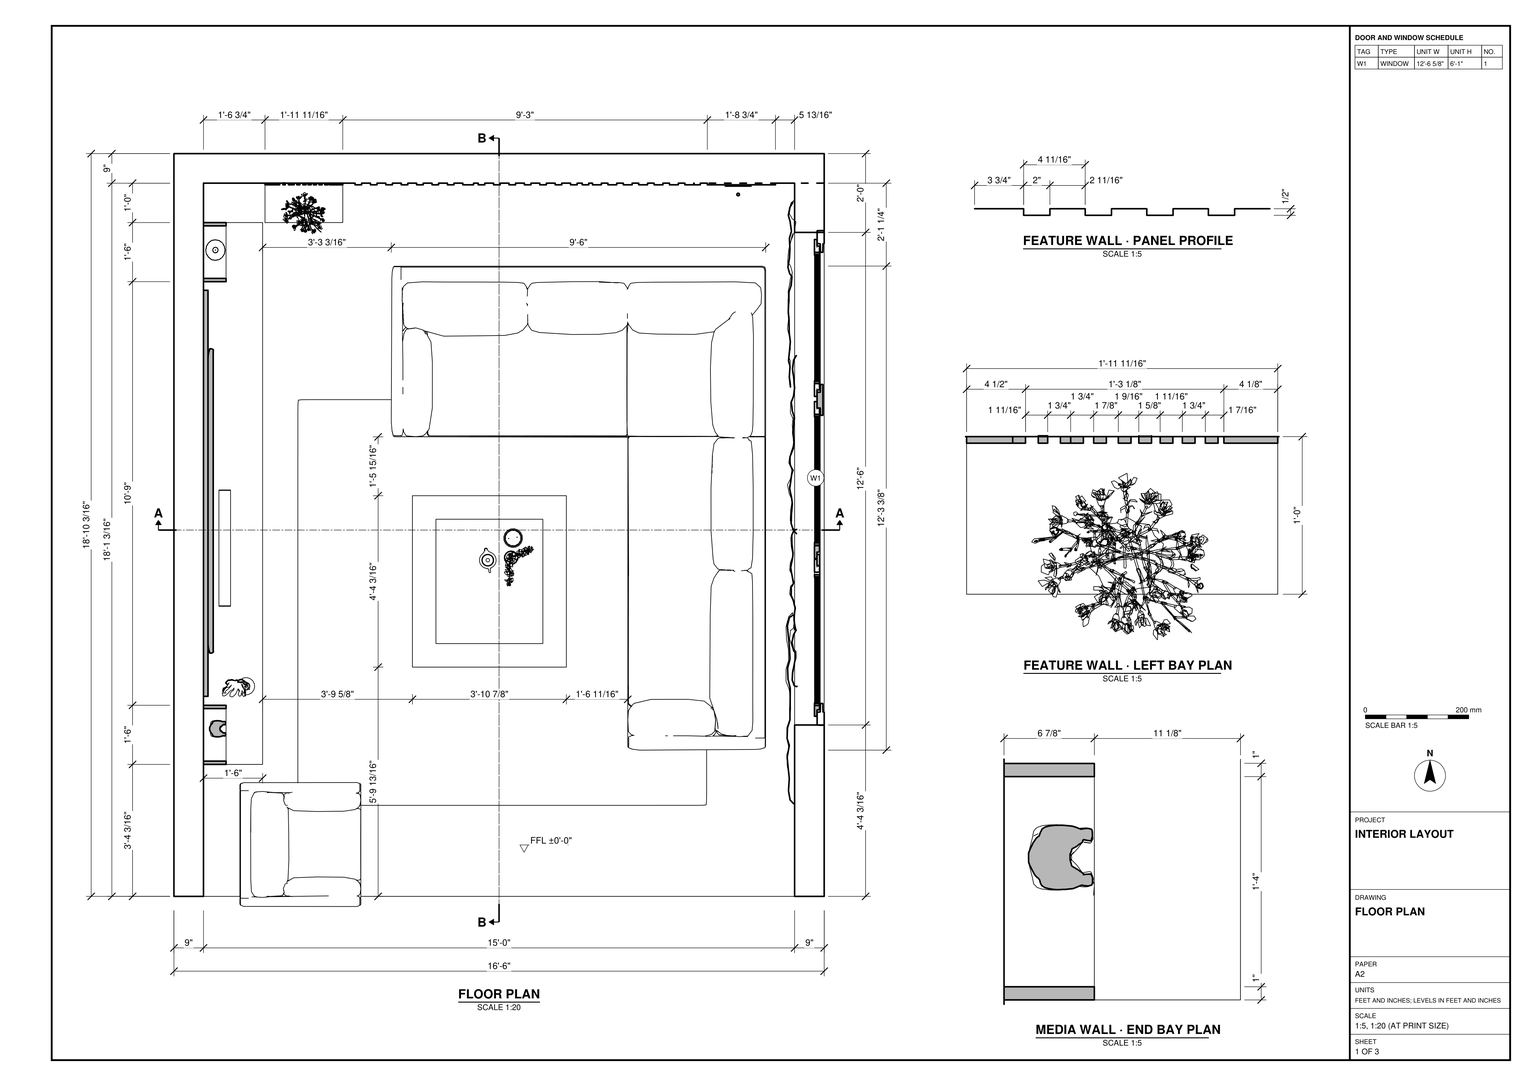
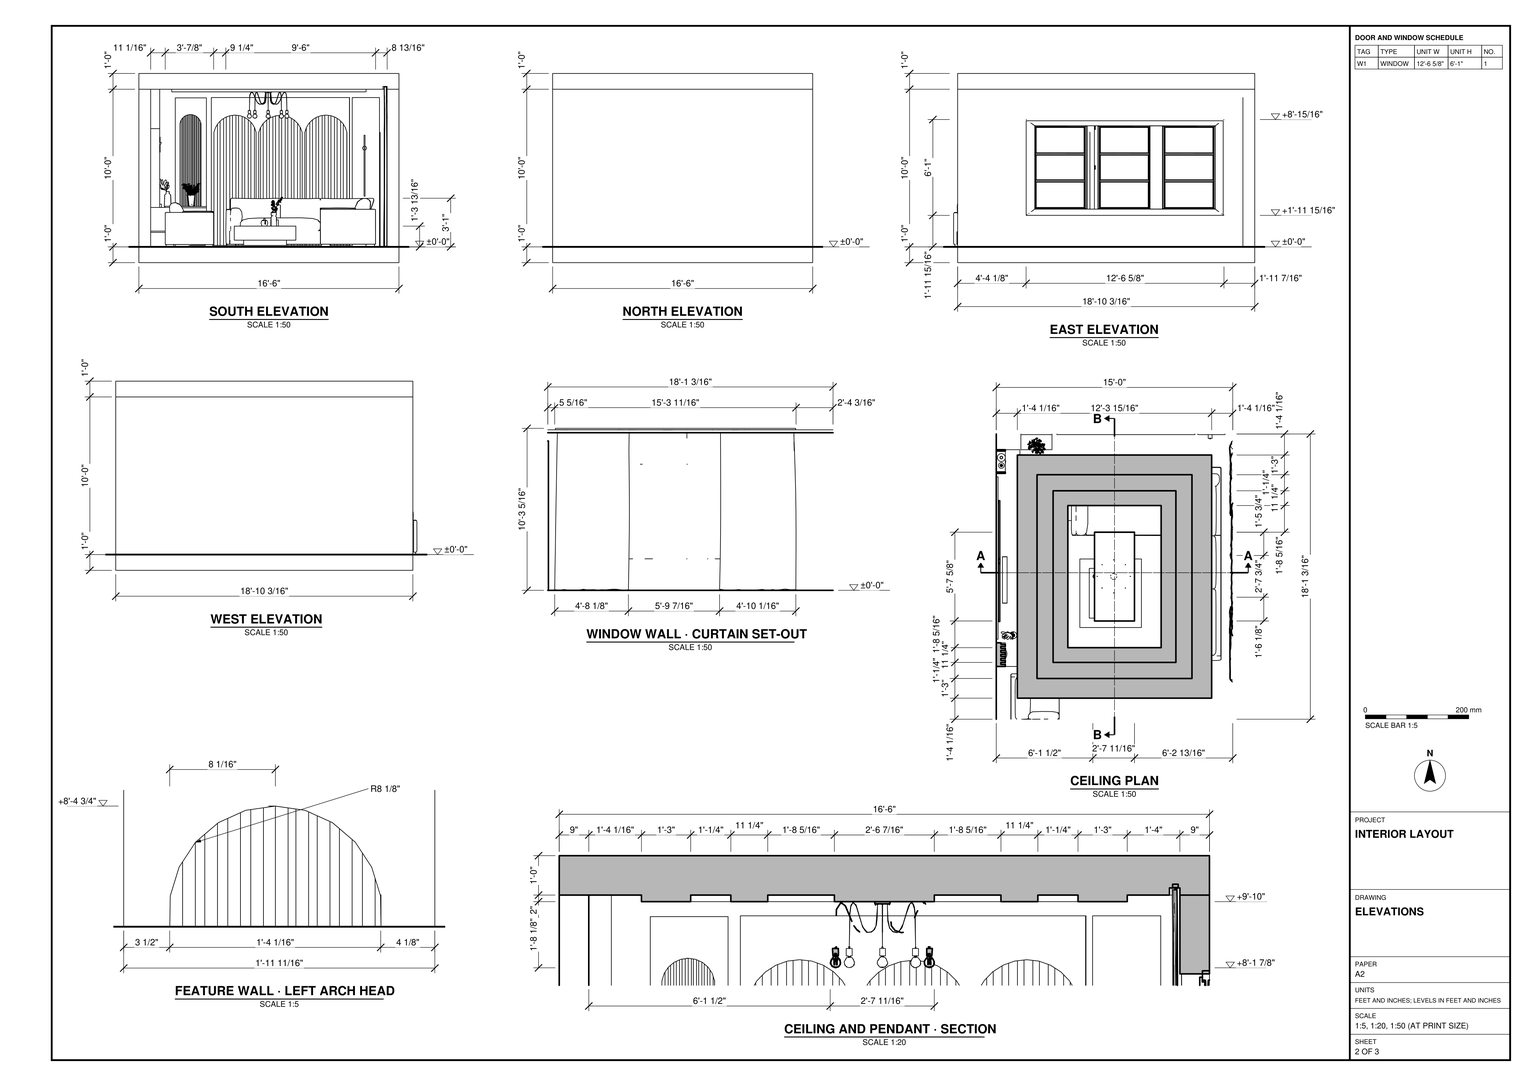
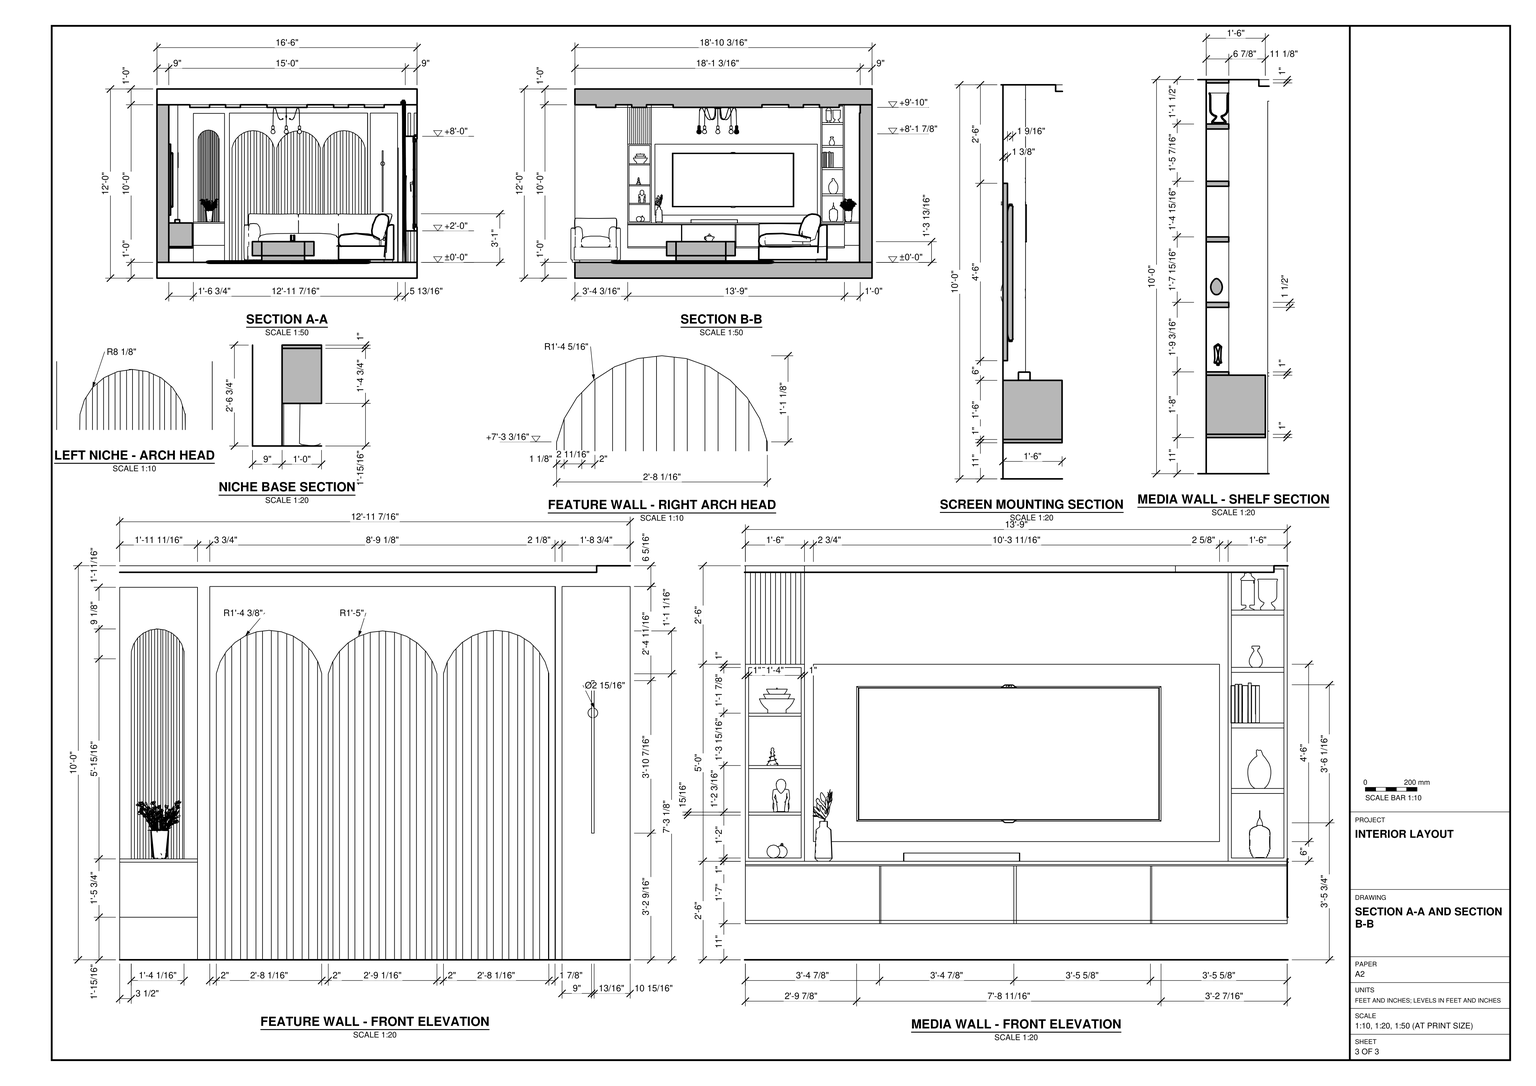
Build the furnished living room shown in task_files/diagram_01.pdf. Work in feet and inches. The overall model is 16'-6" wide, 19'-1 1/4" deep and 12'-0" high, with a single finished floor level at ±0'-0". Model the floor and ceiling slabs and the 9" walls on the north, east and west sides. Leave the south side open as drawn. Use the ceiling plan and sections to form the stepped rectangular bands overhead.

On the north wall, model the narrow arched display niche above its base, the three broad arches with vertical ribbing, and the plain end panel. On the west wall, build the low media cabinet with a screen on its backing panel and open shelves at both ends. Fit the divided window into the east wall and place the curtains on its room side.

Arrange the L-shaped sectional along the feature and window walls. Place the coffee table on the rug inside the L, the armchair near the open southwest corner and the pendant above the table. Decor and loose items may be any suitable library components.

Keep the shell elements and each furniture or joinery piece as separate groups or components, and use components for repeated parts. Save one SketchUp model as output_files/living_room_with_feature_and_media_walls.skp.

# SketchUp Ruby script. Lengths in inches.
U = 1.inch
M = Sketchup.active_model
def pt(a) = Geom::Point3d.new(a.map { |v| v * U })
def face(e, loops, mat)
  f = e.add_face(loops[0].map { |a| pt(a) })
  loops[1..].each { |l| e.add_face(l.map { |a| pt(a) }).erase! }
  f.material = f.back_material = mat if mat
  f
end
# faces: each face lists its corners as indices into pts; further lists are holes
def faces(e, pts, list, mat = nil) = list.each { |f| face(e, (f[0].is_a?(Array) ? f : [f]).map { |l| l.map { |i| pts[i] } }, mat) }
# xy, xz, yz: faces in a plane at the given z, y or x. An outline is a flat list of corners, or four numbers for a rectangle; further outlines are holes
def ring(l) = l.size == 4 ? [[l[0], l[1]], [l[2], l[1]], [l[2], l[3]], [l[0], l[3]]] : l.each_slice(2).to_a
def flat(e, list, mat, &to3) = list.each { |f| face(e, (f[0].is_a?(Array) ? f : [f]).map { |l| ring(l).map { |u, v| to3.(u, v) } }, mat) }
def xy(e, z, list, mat = nil) = flat(e, list, mat) { |x, y| [x, y, z] }
def xz(e, y, list, mat = nil) = flat(e, list, mat) { |x, z| [x, y, z] }
def yz(e, x, list, mat = nil) = flat(e, list, mat) { |y, z| [x, y, z] }
def lines(e, pts, list) = list.each { |a, b| e.add_line(pt(pts[a]), pt(pts[b])) }
# prism: a flat outline (further loops are holes) pulled along v
def prism(e, loops, v, mat = nil)
  f = face(e, loops, mat); d = Geom::Vector3d.new(v.map { |x| x * U })
  f.pushpull(f.normal.samedirection?(d) ? d.length : -d.length)
end
def box(e, o, s, mat = nil) = prism(e, [[o, [o[0] + s[0], o[1], o[2]], [o[0] + s[0], o[1] + s[1], o[2]], [o[0], o[1] + s[1], o[2]]]], [0, 0, s[2]], mat)
def at(x, y, z, deg = 0) = Geom::Transformation.translation(pt([x, y, z])) * Geom::Transformation.rotation(ORIGIN, Z_AXIS, deg.degrees)
def axes(o, x, y, z) = Geom::Transformation.new([*x, 0, *y, 0, *z, 0, *pt(o).to_a, 1])
def part(name) = M.definitions.add(name)
# library, detail: a bought-in or finely detailed component or shape, given as its bounding box
def library(name, o, s) = part(name).tap { |d| box(d.entities, o, s) }
def detail(e, o, s) = box(e.add_group.entities, o, s)
def put(e, d, t, mat = nil) = e.add_instance(d, t).tap { |i| i.material = mat if mat }
def group(e, t, mat = nil) = e.add_group.tap { |g| g.transformation = t; g.material = mat if mat }.entities
root = M.entities
M.materials.add("Delta-Grail-185LF-SS").color = [45, 45, 45]
c1 = library("Window 46-31",[-44.57,-2.6,0],[89.14,5.19,59.84])
c2 = library("Curtains 001",[-91.88,-6.87,0.16],[183.71,15.03,109.46])
c3 = library("Fairfax Sectional",[-59.93,-44.96,0],[104.54,100.01,33.05])
c4 = part("Группа\#472")
prism(c4.entities,[[[0.67,0.67,0],[0.73,0.59,0],[0.77,0.5,0],[0.79,0.39,0],[0.77,0.29,0],[0.73,0.2,0],[0.67,0.12,0],[0.59,0.05,0],[0.5,0.01,0],[0.39,0,0],[0.29,0.01,0],[0.2,0.05,0],[0.12,0.12,0],[0.05,0.2,0],[0.01,0.29,0],[0,0.39,0],[0.01,0.5,0],[0.05,0.59,0],[0.12,0.67,0],[0.2,0.73,0],[0.29,0.77,0],[0.39,0.79,0],[0.5,0.77,0],[0.59,0.73,0]]],[0,0,46.46],"Delta-Grail-185LF-SS")
c5 = part("Группа\#471")
prism(c5.entities,[[[2.95,2.79,0.8],[2.95,2.83,0.88],[2.95,2.86,0.97],[2.95,2.89,1.06],[2.95,2.92,1.15],[2.95,2.93,1.24],[2.95,2.95,1.33],[2.95,2.95,1.42],[2.95,2.95,1.52],[2.95,2.95,1.61],[2.95,2.93,1.7],[2.95,2.92,1.79],[2.95,2.9,1.88],[2.95,2.87,1.97],[2.95,2.83,2.06],[2.95,2.79,2.14],[2.95,2.75,2.22],[2.95,2.7,2.3],[2.95,2.65,2.375],[2.95,2.59,2.45],[2.95,2.52,2.52],[2.95,2.46,2.58],[2.95,2.38,2.64],[2.95,2.31,2.69],[2.95,2.23,2.74],[2.95,2.15,2.79],[2.95,2.07,2.83],[2.95,1.98,2.86],[2.95,1.89,2.89],[2.95,1.8,2.92],[2.95,1.71,2.93],[2.95,1.62,2.95],[2.95,1.53,2.95],[2.95,1.43,2.95],[2.95,1.34,2.95],[2.95,1.25,2.93],[2.95,1.16,2.92],[2.95,1.07,2.9],[2.95,0.98,2.87],[2.95,0.89,2.83],[2.95,0.81,2.79],[2.95,0.73,2.75],[2.95,0.65,2.7],[2.95,0.58,2.65],[2.95,0.5,2.59],[2.95,0.4375,2.52],[2.95,0.37,2.46],[2.95,0.3125,2.38],[2.95,0.26,2.31],[2.95,0.21,2.23],[2.95,0.16,2.15],[2.95,0.12,2.07],[2.95,0.09,1.98],[2.95,0.06,1.89],[2.95,0.04,1.8],[2.95,0.02,1.71],[2.95,0.01,1.62],[2.95,0,1.53],[2.95,0,1.43],[2.95,0.01,1.34],[2.95,0.02,1.25],[2.95,0.03,1.16],[2.95,0.06,1.07],[2.95,0.08,0.98],[2.95,0.12,0.89],[2.95,0.16,0.81],[2.95,0.2,0.73],[2.95,0.25,0.65],[2.95,0.31,0.58],[2.95,0.36,0.5],[2.95,0.43,0.4375],[2.95,0.5,0.37],[2.95,0.57,0.3125],[2.95,0.64,0.26],[2.95,0.72,0.21],[2.95,0.8,0.16],[2.95,0.88,0.12],[2.95,0.97,0.09],[2.95,1.06,0.06],[2.95,1.15,0.04],[2.95,1.24,0.02],[2.95,1.33,0.01],[2.95,1.42,0],[2.95,1.52,0],[2.95,1.61,0.01],[2.95,1.7,0.02],[2.95,1.79,0.03],[2.95,1.88,0.06],[2.95,1.97,0.08],[2.95,2.06,0.12],[2.95,2.14,0.16],[2.95,2.22,0.2],[2.95,2.3,0.25],[2.95,2.375,0.31],[2.95,2.45,0.36],[2.95,2.52,0.43],[2.95,2.58,0.5],[2.95,2.64,0.57],[2.95,2.69,0.64],[2.95,2.74,0.72]]],[-2.95,0,0],"Delta-Grail-185LF-SS")
c6 = part("KEMMA WALL L")
put(c6.entities,c4,at(0,1.08,0))
put(c6.entities,c5,at(0.39,0,35.14))
c7 = part("Группа\#357")
xy(c7.entities,0,[[0,0,118.11,15.75]])
c8 = part("Группа\#473")
put(c8.entities,c7,axes([0,7.84,0],[0,0,0.39176],[0,-0.25,0],[-1,0,0]))
put(c8.entities,c7,axes([0,0,0],[0,0,0.39176],[0,0.25,0],[1,0,0]))
c9 = part("Kemma wall")
put(c9.entities,c6,at(0,2.44,3.71))
put(c9.entities,c8,axes([2.95,0,0],[1,0,0],[0,1,0],[0,0,1.16295]))
c10 = library("Rug 293 007",[-90.2,-61.78,-0.71],[180.4,123.56,1.82])
c11 = library("Fairfax Chair",[-18.9,-18.43,0],[37.75,36.85,33.69])
c12 = library("TV Speaker 002",[-17.72,-1.77,0],[35.44,3.54,2.52])
c13 = library("download?mid=50c7180b9fccec56d493bfe20f94b6ab&ctyp=sp&cv=p8.",[149.43,43.83,17.86],[74.75,0.57,42.04])
c14 = library("Books 53-03",[-4.33,-4.86,0],[8.66,9.72,12.21])
c15 = library("Perfume 101 020",[-1.72,-1.72,-0.02],[3.44,3.44,5.4])
c16 = library("Perfume 101 004",[-2,-2,-0.02],[4,4,6.5])
c17 = library("Interior Props 221 031",[-3.74,-3.52,-0.04],[7.48,7.03,11.78])
c18 = library("Christmas Props 155 013 03",[-3.17,-3,-0.07],[6.8,6.18,4.48])
c19 = library("Interior Props 160 010",[-8.82,-8.31,0],[17.47,16.43,22.13])
c20 = library("Decorative Jar 83-09",[-5.58,-3.02,0],[11.21,6.04,13.74])
c21 = library("Fountain 108-01",[-21.4375,-21.4375,0],[42.875,42.875,30.71])
c22 = library("Decorative Jar 002",[-4.66,-4.66,0.02],[9.32,9.32,23.26])
c23 = library("Vase 007",[-9.22,-3.28,0],[11.85,5.91,21.89])
c24 = library("Interior Props 221 010",[-4.44,-3.51,-0.03],[8.89,7.03,15.76])
c25 = library("Vase 004",[-7.23,-6.39,-0.02],[13.74,12.68,17.81])
c26 = library("Pendant 81-14",[-15.9,-15.86,-20.15],[31.7,31.76,20.15])
xy(root,-12,[[0,0,198,226.1875]])
xy(root,0,[[0,0,9,0,9,217.1875,55.15,217.1875,55.15,216.6875,57.15,216.6875,57.15,217.1875,59.84,217.1875,59.84,216.6875,61.84,216.6875,61.84,217.1875,64.53,217.1875,64.53,216.6875,66.53,216.6875,66.53,217.1875,69.21,217.1875,69.21,216.6875,71.21,216.6875,71.21,217.1875,73.9,217.1875,73.9,216.6875,75.9,216.6875,75.9,217.1875,78.59,217.1875,78.59,216.6875,80.59,216.6875,80.59,217.1875,83.28,217.1875,83.28,216.6875,85.28,216.6875,85.28,217.1875,87.96,217.1875,87.96,216.6875,91.23,216.6875,91.23,217.1875,92.65,217.1875,92.65,216.6875,94.65,216.6875,94.65,217.1875,97.34,217.1875,97.34,216.6875,99.34,216.6875,99.34,217.1875,102.03,217.1875,102.03,216.6875,104.03,216.6875,104.03,217.1875,106.71,217.1875,106.71,216.6875,108.71,216.6875,108.71,217.1875,111.4,217.1875,111.4,216.6875,113.4,216.6875,113.4,217.1875,116.09,217.1875,116.09,216.6875,118.09,216.6875,118.09,217.1875,120.78,217.1875,120.78,216.6875,122.78,216.6875,122.78,217.1875,124.32,217.1875,124.32,216.6875,126.32,216.6875,126.32,217.1875,127.46,217.1875,127.46,216.6875,130.15,216.6875,130.15,217.1875,132.15,217.1875,132.15,216.6875,134.84,216.6875,134.84,217.1875,136.84,217.1875,136.84,216.6875,139.53,216.6875,139.53,217.1875,141.53,217.1875,141.53,216.6875,144.21,216.6875,144.21,217.1875,146.21,217.1875,146.21,216.6875,148.9,216.6875,148.9,217.1875,150.9,217.1875,150.9,216.6875,153.59,216.6875,153.59,217.1875,155.59,217.1875,155.59,216.6875,158.28,216.6875,158.28,217.1875,158.4,217.1875,158.4,216.6875,160.28,216.6875,160.28,217.1875,162.42,217.1875,162.42,216.6875,183.17,216.6875,183.17,217.1875,189,217.1875,189,0,198,0,198,226.1875,0,226.1875],[9,0,189,0,189,217.1875,183.17,217.1875,183.17,216.6875,162.42,216.6875,162.42,217.1875,160.28,217.1875,160.28,216.6875,158.4,216.6875,158.4,217.1875,158.28,217.1875,158.28,216.6875,155.59,216.6875,155.59,217.1875,153.59,217.1875,153.59,216.6875,150.9,216.6875,150.9,217.1875,148.9,217.1875,148.9,216.6875,146.21,216.6875,146.21,217.1875,144.21,217.1875,144.21,216.6875,141.53,216.6875,141.53,217.1875,139.53,217.1875,139.53,216.6875,136.84,216.6875,136.84,217.1875,134.84,217.1875,134.84,216.6875,132.15,216.6875,132.15,217.1875,130.15,217.1875,130.15,216.6875,127.46,216.6875,127.46,217.1875,126.32,217.1875,126.32,216.6875,124.32,216.6875,124.32,217.1875,122.78,217.1875,122.78,216.6875,120.78,216.6875,120.78,217.1875,118.09,217.1875,118.09,216.6875,116.09,216.6875,116.09,217.1875,113.4,217.1875,113.4,216.6875,111.4,216.6875,111.4,217.1875,108.71,217.1875,108.71,216.6875,106.71,216.6875,106.71,217.1875,104.03,217.1875,104.03,216.6875,102.03,216.6875,102.03,217.1875,99.34,217.1875,99.34,216.6875,97.34,216.6875,97.34,217.1875,94.65,217.1875,94.65,216.6875,92.65,216.6875,92.65,217.1875,91.23,217.1875,91.23,216.6875,87.96,216.6875,87.96,217.1875,85.28,217.1875,85.28,216.6875,83.28,216.6875,83.28,217.1875,80.59,217.1875,80.59,216.6875,78.59,216.6875,78.59,217.1875,75.9,217.1875,75.9,216.6875,73.9,216.6875,73.9,217.1875,71.21,217.1875,71.21,216.6875,69.21,216.6875,69.21,217.1875,66.53,217.1875,66.53,216.6875,64.53,216.6875,64.53,217.1875,61.84,217.1875,61.84,216.6875,59.84,216.6875,59.84,217.1875,57.15,217.1875,57.15,216.6875,55.15,216.6875,55.15,217.1875,9,217.1875]])
xy(root,1.1,[[79.78,76.97,112.34,114.85]])
xy(root,5.1,[[[72.62,69.81,119.5,122.01],[79.78,76.97,112.34,114.85]],[79.78,76.97,112.34,114.85]])
xy(root,11,[[9,40.1875,27,205.1875]])
xy(root,12,[[9,40.1875,27,205.1875]])
xy(root,12.97,[[27.73,205.1875,51.42,217.1875]])
xy(root,15.79,[[[72.62,69.81,119.5,122.01],[79.78,76.97,112.34,114.85]],[79.78,76.97,112.34,114.85]])
xy(root,24,[[189,52.1875,198,202.1875]])
xy(root,29.72,[[27.73,205.1875,51.42,217.1875]])
xy(root,30,[[15.875,40.1875,27,40.1875,27,205.1875,15.875,205.1875,15.875,187.1875,9,187.1875,9,58.1875,15.875,58.1875],[9,40.1875,15.875,58.1875],[9,187.1875,15.875,205.1875]])
xy(root,30.72,[[27.73,205.1875,51.42,205.1875,51.42,216.6875,47.31,216.6875,47.31,217.1875,46.87,217.1875,46.87,216.6875,45.9,216.6875,45.9,217.1875,45.12,217.1875,45.12,216.6875,44.15,216.6875,44.15,217.1875,43.43,217.1875,43.43,216.6875,42.46,216.6875,42.46,217.1875,41.81,217.1875,41.81,216.6875,40.84,216.6875,40.84,217.1875,40.24,217.1875,40.24,216.6875,39.28,216.6875,39.28,217.1875,38.37,217.1875,38.37,216.6875,37.4,216.6875,37.4,217.1875,36.62,217.1875,36.62,216.6875,34.87,216.6875,34.87,217.1875,33.9,217.1875,33.9,216.6875,33.18,216.6875,33.18,217.1875,32.21,217.1875,32.21,216.6875,27.73,216.6875],[27.73,216.6875,31.24,217.1875],[31.24,216.6875,32.21,217.1875],[33.18,216.6875,33.9,217.1875],[34.87,216.6875,35.65,217.1875],
  [35.65,216.6875,36.62,217.1875],[37.4,216.6875,38.37,217.1875],[39.28,216.6875,40.24,217.1875],[40.84,216.6875,41.81,217.1875],[42.46,216.6875,43.43,217.1875],
  [44.15,216.6875,45.12,217.1875],[45.9,216.6875,46.87,217.1875],[47.31,216.6875,51.42,217.1875],[33.18,217.1875,33.9,217.25],[40.84,217.1875,41.81,217.25]])
xy(root,31,[[9,41.1875,15.875,57.1875],[9,188.1875,15.875,204.1875]])
xy(root,36,[[9,60.91,10.375,184.5625]])
xy(root,44.05,[[9,41.1875,15.875,57.1875]])
xy(root,44.98,[[9,41.1875,15.875,57.1875]])
xy(root,50.65,[[9,188.1875,15.875,204.1875]])
xy(root,52.17,[[9,188.1875,15.875,204.1875]])
xy(root,58.23,[[9,41.1875,15.875,57.1875]])
xy(root,59.16,[[9,41.1875,15.875,57.1875]])
xy(root,70.59,[[9,188.1875,15.875,204.1875]])
xy(root,72.11,[[9,188.1875,15.875,204.1875]])
xy(root,74.17,[[9,41.1875,15.875,57.1875]])
xy(root,75.1,[[9,41.1875,15.875,57.1875]])
xy(root,87.53,[[9,188.1875,15.875,204.1875]])
xy(root,89,[[9,41.1875,15.875,57.1875]])
xy(root,89.05,[[9,188.1875,15.875,204.1875]])
xy(root,90,[[9,40.1875,15.875,40.1875,15.875,41.74,12.5,41.74,12.5,43.25,15.875,43.25,15.875,44.81,12.5,44.81,12.5,46.3125,15.875,46.3125,15.875,47.87,12.5,47.87,12.5,49.375,15.875,49.375,15.875,50.93,12.5,50.93,12.5,52.4375,15.875,52.4375,15.875,53.99,12.5,53.99,12.5,55.5,15.875,55.5,15.875,57.06,12.5,57.06,12.5,58.1875,9,58.1875],[12.5,41.74,15.875,43.25],[12.5,44.81,15.875,46.3125],[12.5,47.87,15.875,49.375],[12.5,50.93,15.875,52.4375],
  [12.5,53.99,15.875,55.5],[12.5,57.06,15.875,58.1875],[9,60.91,10.375,184.5625]])
xy(root,96,[[189,52.1875,198,202.1875]])
xy(root,104.97,[[9,188.1875,15.875,204.1875]])
xy(root,106.49,[[9,188.1875,15.875,204.1875]])
xy(root,113.4375,[[27.73,216.6875,51.42,217.1875]])
xy(root,113.6875,[[55.15,216.6875,160.28,217.1875],[162.42,216.6875,183.17,217.1875]])
xy(root,118,[[[25.04,16.04,172.96,201.15],[40.03,31.03,157.97,186.16]],[[52.26,43.26,145.74,173.93],[63.49,54.49,134.51,162.69]],[83.79,74.79,114.21,142.4]])
xy(root,119,[[9,188.1875,15.875,204.1875]])
xy(root,120,[[0,0,0,226.1875,198,226.1875,198,0,189,0,189,217.1875,9,217.1875,9,0],[[9,0,9,40.1875,15.875,40.1875,15.875,41.74,12.5,41.74,12.5,43.25,15.875,43.25,15.875,44.81,12.5,44.81,12.5,46.3125,15.875,46.3125,15.875,47.87,12.5,47.87,12.5,49.375,15.875,49.375,15.875,50.93,12.5,50.93,12.5,52.4375,15.875,52.4375,15.875,53.99,12.5,53.99,12.5,55.5,15.875,55.5,15.875,57.06,12.5,57.06,12.5,58.1875,9,58.1875,9,187.1875,15.875,187.1875,15.875,205.1875,9,205.1875,9,217.1875,185.8125,217.1875,185.8125,0],[25.04,16.04,172.96,201.15]],[[40.03,31.03,157.97,186.16],[52.26,43.26,145.74,173.93]],[9,40.1875,9,58.1875,12.5,58.1875,12.5,57.06,15.875,57.06,15.875,55.5,12.5,55.5,12.5,53.99,15.875,53.99,15.875,52.4375,12.5,52.4375,12.5,50.93,15.875,50.93,15.875,49.375,12.5,49.375,12.5,47.87,15.875,47.87,15.875,46.3125,12.5,46.3125,12.5,44.81,15.875,44.81,15.875,43.25,12.5,43.25,12.5,41.74,15.875,41.74,15.875,40.1875],[[63.49,54.49,134.51,162.69],[83.79,74.79,114.21,142.4]],
  [9,187.1875,15.875,205.1875]])
xy(root,122.1875,[[185.8125,0,189,217.1875]])
xy(root,132,[[0,0,198,226.1875]])
xz(root,0,[[0,-12,198,0],[0,0,9,120],[189,0,198,120],[0,120,185.8125,120,185.8125,122.1875,189,122.1875,189,120,198,120,198,132,0,132]])
xz(root,16.04,[[25.04,118,172.96,120]])
xz(root,31.03,[[40.03,118,157.97,120]])
xz(root,40.1875,[[9,11,27,12],[9,12,27,30],[9,30,15.875,90],[9,90,15.875,120]])
xz(root,41.1875,[[9,31,15.875,44.05],[9,44.05,15.875,44.98],[9,44.98,15.875,58.23],[9,58.23,15.875,59.16],[9,59.16,15.875,74.17],
  [9,74.17,15.875,75.1],[9,75.1,15.875,89]])
xz(root,41.74,[[12.5,90,15.875,120]])
xz(root,43.25,[[12.5,90,15.875,120]])
xz(root,43.26,[[52.26,118,145.74,120]])
xz(root,44.81,[[12.5,90,15.875,120]])
xz(root,46.3125,[[12.5,90,15.875,120]])
xz(root,47.87,[[12.5,90,15.875,120]])
xz(root,49.375,[[12.5,90,15.875,120]])
xz(root,50.93,[[12.5,90,15.875,120]])
xz(root,52.1875,[[189,24,198,96]])
xz(root,52.4375,[[12.5,90,15.875,120]])
xz(root,53.99,[[12.5,90,15.875,120]])
xz(root,54.49,[[63.49,118,134.51,120]])
xz(root,55.5,[[12.5,90,15.875,120]])
xz(root,57.06,[[12.5,90,15.875,120]])
xz(root,57.1875,[[9,31,15.875,44.05],[9,44.05,15.875,44.98],[9,44.98,15.875,58.23],[9,58.23,15.875,59.16],[9,59.16,15.875,74.17],
  [9,74.17,15.875,75.1],[9,75.1,15.875,89]])
xz(root,58.1875,[[9,30,15.875,90],[9,90,12.5,120]])
xz(root,60.91,[[9,36,10.375,90]])
xz(root,69.81,[[72.62,5.1,119.5,15.79]])
xz(root,74.79,[[83.79,118,114.21,120]])
xz(root,76.97,[[79.78,1.1,112.34,5.1],[79.78,5.1,112.34,15.79]])
xz(root,114.85,[[79.78,1.1,112.34,5.1],[79.78,5.1,112.34,15.79]])
xz(root,122.01,[[72.62,5.1,119.5,15.79]])
xz(root,142.4,[[83.79,118,114.21,120]])
xz(root,162.69,[[63.49,118,134.51,120]])
xz(root,173.93,[[52.26,118,145.74,120]])
xz(root,184.5625,[[9,36,10.375,90]])
xz(root,186.16,[[40.03,118,157.97,120]])
xz(root,187.1875,[[9,30,15.875,120]])
xz(root,188.1875,[[9,31,15.875,50.65],[9,50.65,15.875,52.17],[9,52.17,15.875,70.59],[9,70.59,15.875,72.11],[9,72.11,15.875,87.53],
  [9,87.53,15.875,89.05],[9,89.05,15.875,104.97],[9,104.97,15.875,106.49],[9,106.49,15.875,119]])
xz(root,201.15,[[25.04,118,172.96,120]])
xz(root,202.1875,[[189,24,198,96]])
xz(root,204.1875,[[9,31,15.875,50.65],[9,50.65,15.875,52.17],[9,52.17,15.875,70.59],[9,70.59,15.875,72.11],[9,72.11,15.875,87.53],
  [9,87.53,15.875,89.05],[9,89.05,15.875,104.97],[9,104.97,15.875,106.49],[9,106.49,15.875,119]])
xz(root,205.1875,[[9,11,27,12],[9,12,27,30],[27.73,12.97,51.42,29.72],[27.73,29.72,51.42,30.72],[9,30,15.875,120]])
xz(root,216.6875,[[55.15,0,57.15,0,57.15,87.2,58.3,90.75,59.84,93.3,60.23,93.95,61.84,95.61,62.83,96.63,64.53,97.72,65.97,98.65,66.53,98.85,69.21,99.81,69.48,99.9,71.21,100.1,73.19,100.33,73.9,100.25,75.9,100.02,76.9,99.9,78.59,99.3,80.42,98.65,80.59,98.54,83.28,96.81,83.56,96.63,85.28,94.86,86.16,93.95,88.08,90.75,89.23,87.2,89.23,0,91.23,0,91.23,87.09,92.51,90.65,92.65,90.86,94.55,93.84,94.65,93.9375,97.24,96.49,97.34,96.56,99.34,97.8,100.45,98.49,102.03,99.04,104.02,99.73,104.03,99.73,106.71,100.03,107.78,100.15,108.71,100.05,111.4,99.75,111.53,99.73,113.4,99.08,115.11,98.49,116.09,97.88,118.09,96.63,118.32,96.49,120.78,94.06,121,93.84,122.78,91.06,123.04,90.65,124.32,87.09,124.32,0,126.32,0,126.32,87.2,127.46,90.74,127.47,90.75,129.4,93.95,130.15,94.73,132,96.63,132.15,96.73,134.84,98.46,135.14,98.65,136.84,99.26,138.65,99.9,139.53,100,141.53,100.23,142.36,100.33,144.21,100.12,146.07,99.9,146.21,99.85,148.9,98.89,149.58,98.65,150.9,97.8,152.72,96.63,153.59,95.74,155.32,93.95,155.59,93.51,157.25,90.75,158.28,87.59,158.4,87.2,158.4,0,160.28,0,160.28,113.6875,55.15,113.6875],[59.84,0,61.84,0,61.84,95.61,60.23,93.95,59.84,93.3],[64.53,0,66.53,0,66.53,98.85,65.97,98.65,64.53,97.72],[69.21,0,71.21,0,71.21,100.1,69.48,99.9,69.21,99.81],[73.9,0,75.9,0,75.9,100.02,73.9,100.25],
  [78.59,0,80.59,0,80.59,98.54,80.42,98.65,78.59,99.3],[83.28,0,85.28,0,85.28,94.86,83.56,96.63,83.28,96.81],[87.96,0,89.23,0,89.23,87.2,88.08,90.75,87.96,90.95],[92.65,0,94.65,0,94.65,93.9375,94.55,93.84,92.65,90.86],[97.34,0,99.34,0,99.34,97.8,97.34,96.56],
  [102.03,0,104.03,0,104.03,99.73,104.02,99.73,102.03,99.04],[106.71,0,108.71,0,108.71,100.05,107.78,100.15,106.71,100.03],[111.4,0,113.4,0,113.4,99.08,111.53,99.73,111.4,99.75],[116.09,0,118.09,0,118.09,96.63,116.09,97.88],[120.78,0,122.78,0,122.78,91.06,121,93.84,120.78,94.06],
  [127.46,0,130.15,0,130.15,94.73,129.4,93.95,127.47,90.75,127.46,90.74],[132.15,0,134.84,0,134.84,98.46,132.15,96.73],[136.84,0,139.53,0,139.53,100,138.65,99.9,136.84,99.26],[141.53,0,144.21,0,144.21,100.12,142.36,100.33,141.53,100.23],[146.21,0,148.9,0,148.9,98.89,146.21,99.85],
  [150.9,0,153.59,0,153.59,95.74,152.72,96.63,150.9,97.8],[155.59,0,158.28,0,158.28,87.59,157.25,90.75,155.59,93.51],[162.42,0,183.17,113.6875],[27.73,30.72,31.24,30.72,31.24,91.64,31.27,93.93,31.95,96.11,32.21,96.52,33.18,97.99,33.2,98.02,33.9,98.62,34.87,99.44,34.94,99.5,35.65,99.82,36.62,100.26,37.02,100.4375,37.4,100.49,39.28,100.76,40.24,100.62,40.84,100.54,41.54,100.4375,41.81,100.32,42.46,100.02,43.43,99.58,43.62,99.5,44.15,99.04,45.12,98.22,45.35,98.02,45.9,97.18,46.61,96.11,46.87,95.26,47.28,93.93,47.31,91.64,47.31,30.72,51.42,30.72,51.42,113.4375,27.73,113.4375],[31.24,30.72,32.21,30.72,32.21,96.52,31.95,96.11,31.27,93.93,31.24,91.64],
  [33.18,30.72,33.9,30.72,33.9,98.62,33.2,98.02,33.18,97.99],[34.87,30.72,35.65,30.72,35.65,99.82,34.94,99.5,34.87,99.44],[35.65,30.72,36.62,30.72,36.62,100.26,35.65,99.82],[37.4,30.72,38.37,30.72,38.37,100.62,38.34,100.625,37.4,100.49],[39.28,30.72,40.24,30.72,40.24,100.62,39.28,100.76],
  [40.84,30.72,41.81,30.72,41.81,100.32,41.54,100.4375,40.84,100.54],[42.46,30.72,43.43,30.72,43.43,99.58,42.46,100.02],[44.15,30.72,45.12,30.72,45.12,98.22,44.15,99.04],[45.9,30.72,46.87,30.72,46.87,95.26,46.61,96.11,45.9,97.18]])
xz(root,217.1875,[[9,0,27.73,0,27.73,113.4375,51.42,113.4375,51.42,0,55.15,0,55.15,113.6875,160.4,113.6875,160.4,0,162.42,0,162.42,113.6875,183.17,113.6875,183.17,0,189,0,189,120,9,120],[27.73,0,51.42,12.97],[57.15,0,59.84,0,59.84,93.3,58.3,90.75,57.15,87.2],[61.84,0,64.53,0,64.53,97.72,62.83,96.63,61.84,95.61],[66.53,0,69.21,0,69.21,99.81,66.53,98.85],
  [71.21,0,73.9,0,73.9,100.25,73.19,100.33,71.21,100.1],[75.9,0,78.59,0,78.59,99.3,76.9,99.9,75.9,100.02],[80.59,0,83.28,0,83.28,96.81,80.59,98.54],[85.28,0,87.96,0,87.96,90.95,86.16,93.95,85.28,94.86],[91.23,0,92.65,0,92.65,90.86,92.51,90.65,91.23,87.09],
  [94.65,0,97.34,0,97.34,96.56,97.24,96.49,94.65,93.9375],[99.34,0,102.03,0,102.03,99.04,100.45,98.49,99.34,97.8],[104.03,0,106.71,0,106.71,100.03,104.03,99.73],[108.71,0,111.4,0,111.4,99.75,108.71,100.05],[113.4,0,116.09,0,116.09,97.88,115.11,98.49,113.4,99.08],
  [118.09,0,120.78,0,120.78,94.06,118.32,96.49,118.09,96.63],[122.78,0,124.32,0,124.32,87.09,123.04,90.65,122.78,91.06],[126.32,0,127.46,0,127.46,90.74,126.32,87.2],[130.15,0,132.15,0,132.15,96.73,132,96.63,130.15,94.73],[134.84,0,136.84,0,136.84,99.26,135.14,98.65,134.84,98.46],
  [139.53,0,141.53,0,141.53,100.23,139.53,100],[144.21,0,146.21,0,146.21,99.85,146.07,99.9,144.21,100.12],[148.9,0,150.9,0,150.9,97.8,149.58,98.65,148.9,98.89],[153.59,0,155.59,0,155.59,93.51,155.32,93.95,153.59,95.74],[158.28,0,158.4,0,158.4,87.2,158.28,87.59],
  [160.28,0,160.4,113.6875],[162.96,0,164.96,113.6875],[167.65,0,169.65,113.6875],[172.34,0,174.34,113.6875],[177.03,0,179.03,113.6875],
  [181.71,0,183.17,113.6875],[191.09,0,193.09,113.6875],[195.78,0,197.78,113.6875],[27.73,12.97,51.42,29.72],[27.73,29.72,51.42,30.72],
  [27.73,30.72,27.73,113.4375,51.42,113.4375,51.42,30.72,47.31,30.72,47.31,100.76,31.24,100.76,31.24,30.72],[31.24,30.72,31.24,91.64,31.27,93.93,31.95,96.11,32.21,96.52,32.21,30.72],[32.21,30.72,33.18,30.72,33.18,97.99,32.21,96.52],[33.18,30.72,33.18,97.99,33.2,98.02,33.9,98.62,33.9,30.72],[33.9,30.72,34.87,30.72,34.87,99.44,33.9,98.62],
  [34.87,30.72,34.87,99.44,34.94,99.5,35.65,99.82,35.65,30.72],[35.65,30.72,35.65,99.82,36.62,100.26,36.62,30.72],[36.62,30.72,37.4,30.72,37.4,100.49,37.02,100.4375,36.62,100.26],[37.4,30.72,37.4,100.49,38.34,100.625,38.37,100.62,38.37,30.72],[38.37,30.72,39.28,30.72,39.28,100.76,38.34,100.625,38.37,100.62],
  [39.28,30.72,39.28,100.76,40.24,100.62,40.24,30.72],[40.24,30.72,40.84,30.72,40.84,100.54,40.24,100.62],[40.84,30.72,40.84,100.54,41.54,100.4375,41.81,100.32,41.81,30.72],[41.81,30.72,42.46,30.72,42.46,100.02,41.81,100.32],[42.46,30.72,42.46,100.02,43.43,99.58,43.43,30.72],
  [43.43,30.72,44.15,30.72,44.15,99.04,43.62,99.5,43.43,99.58],[44.15,30.72,44.15,99.04,45.12,98.22,45.12,30.72],[45.12,30.72,45.9,30.72,45.9,97.18,45.35,98.02,45.12,98.22],[45.9,30.72,45.9,97.18,46.61,96.11,46.87,95.26,46.87,30.72],[46.87,30.72,47.31,30.72,47.31,91.64,47.28,93.93,46.87,95.26],
  [185.8125,120,189,122.1875]])
xz(root,217.25,[[33.18,30.72,33.18,97.99,33.2,98.02,33.9,98.62,33.9,30.72]])
xz(root,226.1875,[[0,-12,198,0],[0,0,198,120],[0,120,198,132]])
yz(root,0,[[0,-12,226.1875,0],[0,0,226.1875,120],[0,120,226.1875,132]])
yz(root,9,[[0,0,217.1875,0,217.1875,120,205.1875,120,205.1875,11,40.1875,11,40.1875,120,0,120],[40.1875,11,205.1875,12],[[40.1875,12,205.1875,30],[188.1875,20.84,204.1875,22.36]],[188.1875,20.84,204.1875,22.36],[[40.1875,30,58.1875,90],[41.1875,31,57.1875,89]],
  [[58.1875,30,187.1875,120],[60.91,36,184.5625,90]],[[187.1875,30,205.1875,120],[188.1875,31,204.1875,119]],[41.1875,31,57.1875,44.05],[188.1875,31,204.1875,50.65],[60.91,36,184.5625,90],
  [41.1875,44.05,57.1875,44.98],[41.1875,44.98,57.1875,58.23],[188.1875,50.65,204.1875,52.17],[188.1875,52.17,204.1875,70.59],[41.1875,58.23,57.1875,59.16],
  [41.1875,59.16,57.1875,74.17],[188.1875,70.59,204.1875,72.11],[188.1875,72.11,204.1875,87.53],[41.1875,74.17,57.1875,75.1],[41.1875,75.1,57.1875,89],
  [188.1875,87.53,204.1875,89.05],[188.1875,89.05,204.1875,104.97],[40.1875,90,58.1875,120],[188.1875,104.97,204.1875,106.49],[188.1875,106.49,204.1875,119]])
yz(root,10.375,[[60.91,36,184.5625,90]])
yz(root,12.5,[[41.74,90,43.25,120],[44.81,90,46.3125,120],[47.87,90,49.375,120],[50.93,90,52.4375,120],[53.99,90,55.5,120],
  [57.06,90,58.1875,120]])
yz(root,15.875,[[[40.1875,30,58.1875,90],[41.1875,31,57.1875,89]],[[187.1875,30,205.1875,120],[188.1875,31,204.1875,119]],[41.1875,44.05,57.1875,44.98],[188.1875,50.65,204.1875,52.17],[41.1875,58.23,57.1875,59.16],
  [188.1875,70.59,204.1875,72.11],[41.1875,74.17,57.1875,75.1],[188.1875,87.53,204.1875,89.05],[40.1875,90,41.74,120],[43.25,90,44.81,120],
  [46.3125,90,47.87,120],[49.375,90,50.93,120],[52.4375,90,53.99,120],[55.5,90,57.06,120],[188.1875,104.97,204.1875,106.49]])
yz(root,25.04,[[16.04,118,40.1875,120],[40.1875,118,58.1875,120],[58.1875,118,171.15,120],[171.15,118,201.15,120]])
yz(root,27,[[40.1875,11,81.04,12],[81.04,11,81.4375,12],[81.4375,11,121.9375,12],[121.9375,11,122.6875,12],[122.6875,11,163.54,12],
  [163.54,11,163.9375,12],[163.9375,11,205.1875,12],[40.1875,12,81.04,28.6],[81.04,12,81.4375,28.6],[81.4375,12,121.9375,28.6],
  [121.9375,12,122.6875,28.6],[122.6875,12,163.54,28.6],[163.54,12,163.9375,28.6],[163.9375,12,205.1875,28.6],[40.1875,28.6,205.1875,29],
  [40.1875,29,205.1875,30]])
yz(root,27.73,[[205.1875,12.97,217.1875,29.72],[205.1875,29.72,217.1875,30.72],[216.6875,30.72,217.1875,113.4375]])
yz(root,31.24,[[216.6875,30.72,217.1875,91.64]])
yz(root,32.21,[[216.6875,30.72,217.1875,96.52]])
yz(root,33.18,[[216.6875,30.72,217.1875,97.99],[217.1875,30.72,217.25,97.99]])
yz(root,33.9,[[216.6875,30.72,217.1875,98.62],[217.1875,30.72,217.25,98.62]])
yz(root,34.87,[[216.6875,30.72,217.1875,99.44]])
yz(root,35.65,[[216.6875,30.72,217.1875,99.82]])
yz(root,36.62,[[216.6875,30.72,217.1875,100.26]])
yz(root,37.4,[[216.6875,30.72,217.1875,100.49]])
yz(root,38.37,[[216.6875,30.72,217.1875,100.62]])
yz(root,39.28,[[216.6875,30.72,217.1875,100.76]])
yz(root,40.03,[[31.03,118,40.1875,120],[40.1875,118,58.1875,120],[58.1875,118,171.15,120],[171.15,118,186.16,120]])
yz(root,40.24,[[216.6875,30.72,217.1875,100.62]])
yz(root,40.84,[[216.6875,30.72,217.1875,100.54],[217.1875,30.72,217.25,100.54]])
yz(root,41.81,[[216.6875,30.72,217.1875,100.32],[217.1875,30.72,217.25,100.32]])
yz(root,42.46,[[216.6875,30.72,217.1875,100.02]])
yz(root,43.43,[[216.6875,30.72,217.1875,99.58]])
yz(root,44.15,[[216.6875,30.72,217.1875,99.04]])
yz(root,45.12,[[216.6875,30.72,217.1875,98.22]])
yz(root,45.9,[[216.6875,30.72,217.1875,97.18]])
yz(root,46.87,[[216.6875,30.72,217.1875,95.26]])
yz(root,47.31,[[216.6875,30.72,217.1875,91.64]])
yz(root,51.42,[[205.1875,12.97,217.1875,29.72],[205.1875,29.72,217.1875,30.72],[216.6875,30.72,217.1875,113.4375]])
yz(root,52.26,[[43.26,118,58.1875,120],[58.1875,118,171.15,120],[171.15,118,173.93,120]])
yz(root,55.15,[[216.6875,0,217.1875,113.6875]])
yz(root,57.15,[[216.6875,0,217.1875,87.2]])
yz(root,59.84,[[216.6875,0,217.1875,93.3]])
yz(root,61.84,[[216.6875,0,217.1875,87.2],[216.6875,87.2,217.1875,95.61]])
yz(root,63.49,[[54.49,118,58.1875,120],[58.1875,118,162.69,120]])
yz(root,64.53,[[216.6875,0,217.1875,97.72]])
yz(root,66.53,[[216.6875,0,217.1875,87.2],[216.6875,87.2,217.1875,98.85]])
yz(root,69.21,[[216.6875,0,217.1875,99.81]])
yz(root,71.21,[[216.6875,0,217.1875,87.2],[216.6875,87.2,217.1875,100.1]])
yz(root,72.62,[[69.81,5.1,122.01,15.79]])
yz(root,73.9,[[216.6875,0,217.1875,100.25]])
yz(root,75.9,[[216.6875,0,217.1875,87.2],[216.6875,87.2,217.1875,100.02]])
yz(root,78.59,[[216.6875,0,217.1875,99.3]])
yz(root,79.78,[[76.97,1.1,114.85,5.1],[76.97,5.1,114.85,15.79]])
yz(root,80.59,[[216.6875,0,217.1875,87.2],[216.6875,87.2,217.1875,98.54]])
yz(root,83.28,[[216.6875,0,217.1875,96.81]])
yz(root,83.79,[[74.79,118,142.4,120]])
yz(root,85.28,[[216.6875,0,217.1875,87.2],[216.6875,87.2,217.1875,94.86]])
yz(root,87.96,[[216.6875,0,217.1875,90.95]])
yz(root,91.23,[[216.6875,0,217.1875,87.09]])
yz(root,92.65,[[216.6875,0,217.1875,90.86]])
yz(root,94.65,[[216.6875,0,217.1875,87.2],[216.6875,87.2,217.1875,93.9375]])
yz(root,97.34,[[216.6875,0,217.1875,96.56]])
yz(root,99.34,[[216.6875,0,217.1875,87.2],[216.6875,87.2,217.1875,97.8]])
yz(root,102.03,[[216.6875,0,217.1875,99.04]])
yz(root,104.03,[[216.6875,0,217.1875,87.2],[216.6875,87.2,217.1875,99.73]])
yz(root,106.71,[[216.6875,0,217.1875,100.03]])
yz(root,108.71,[[216.6875,0,217.1875,87.2],[216.6875,87.2,217.1875,100.05]])
yz(root,111.4,[[216.6875,0,217.1875,99.75]])
yz(root,112.34,[[76.97,1.1,114.85,5.1],[76.97,5.1,114.85,15.79]])
yz(root,113.4,[[216.6875,0,217.1875,87.2],[216.6875,87.2,217.1875,99.08]])
yz(root,114.21,[[74.79,118,142.4,120]])
yz(root,116.09,[[216.6875,0,217.1875,97.88]])
yz(root,118.09,[[216.6875,0,217.1875,87.2],[216.6875,87.2,217.1875,96.63]])
yz(root,119.5,[[69.81,5.1,122.01,15.79]])
yz(root,120.78,[[216.6875,0,217.1875,94.06]])
yz(root,122.78,[[216.6875,0,217.1875,87.2],[216.6875,87.2,217.1875,91.06]])
yz(root,124.32,[[216.6875,0,217.1875,87.09]])
yz(root,126.32,[[216.6875,0,217.1875,87.2]])
yz(root,127.46,[[216.6875,0,217.1875,87.2],[216.6875,87.2,217.1875,90.74]])
yz(root,130.15,[[216.6875,0,217.1875,94.73]])
yz(root,132.15,[[216.6875,0,217.1875,87.2],[216.6875,87.2,217.1875,96.73]])
yz(root,134.51,[[54.49,118,162.69,120]])
yz(root,134.84,[[216.6875,0,217.1875,98.46]])
yz(root,136.84,[[216.6875,0,217.1875,87.2],[216.6875,87.2,217.1875,99.26]])
yz(root,139.53,[[216.6875,0,217.1875,100]])
yz(root,141.53,[[216.6875,0,217.1875,87.2],[216.6875,87.2,217.1875,100.23]])
yz(root,144.21,[[216.6875,0,217.1875,100.12]])
yz(root,145.74,[[43.26,118,173.93,120]])
yz(root,146.21,[[216.6875,0,217.1875,87.2],[216.6875,87.2,217.1875,99.85]])
yz(root,148.9,[[216.6875,0,217.1875,98.89]])
yz(root,150.9,[[216.6875,0,217.1875,87.2],[216.6875,87.2,217.1875,97.8]])
yz(root,153.59,[[216.6875,0,217.1875,95.74]])
yz(root,155.59,[[216.6875,0,217.1875,87.2],[216.6875,87.2,217.1875,93.51]])
yz(root,157.97,[[31.03,118,186.16,120]])
yz(root,158.28,[[216.6875,0,217.1875,87.59]])
yz(root,158.4,[[216.6875,0,217.1875,87.2]])
yz(root,160.28,[[216.6875,0,217.1875,87.2],[216.6875,87.2,217.1875,113.6875]])
yz(root,162.42,[[216.6875,0,217.1875,113.6875]])
yz(root,172.96,[[16.04,118,201.15,120]])
yz(root,183.17,[[216.6875,0,217.1875,113.6875]])
yz(root,185.8125,[[0,120,217.1875,122.1875]])
yz(root,189,[[[0,0,217.1875,120],[52.1875,24,202.1875,96]],[0,120,217.1875,122.1875]])
yz(root,198,[[0,-12,226.1875,0],[[0,0,226.1875,120],[52.1875,24,202.1875,96]],[0,120,226.1875,132]])
p = [[91.23,217.1875,87.09],[92.51,217.1875,90.65],[92.51,216.6875,90.65],[91.23,216.6875,87.09],[123.04,217.1875,90.65],[124.32,217.1875,87.09],
  [124.32,216.6875,87.09],[123.04,216.6875,90.65],[57.15,217.1875,87.2],[58.3,217.1875,90.75],[58.3,216.6875,90.75],[57.15,216.6875,87.2],
  [126.32,217.1875,87.2],[127.46,217.1875,90.74],[127.46,216.6875,90.74],[126.32,216.6875,87.2],[158.28,217.1875,87.59],[158.4,217.1875,87.2],
  [158.4,216.6875,87.2],[158.28,216.6875,87.59],[92.65,217.1875,90.86],[92.65,216.6875,90.86],[122.78,217.1875,91.06],[122.78,216.6875,91.06],
  [59.84,217.1875,93.3],[59.84,216.6875,93.3],[86.16,217.1875,93.95],[87.96,217.1875,90.95],[87.96,216.6875,90.95],[86.16,216.6875,93.95],
  [31.27,217.1875,93.93],[31.24,217.1875,91.64],[31.24,216.6875,91.64],[31.27,216.6875,93.93],[47.28,217.1875,93.93],[47.31,217.1875,91.64],
  [47.31,216.6875,91.64],[47.28,216.6875,93.93],[155.32,217.1875,93.95],[155.59,217.1875,93.51],[155.59,216.6875,93.51],[155.32,216.6875,93.95],
  [31.95,217.1875,96.11],[31.95,216.6875,96.11],[46.87,217.1875,95.26],[46.87,216.6875,95.26],[94.65,217.1875,93.9375],[97.24,217.1875,96.49],
  [97.24,216.6875,96.49],[94.65,216.6875,93.9375],[85.28,217.1875,94.86],[85.28,216.6875,94.86],[153.59,217.1875,95.74],[153.59,216.6875,95.74],
  [118.32,217.1875,96.49],[120.78,217.1875,94.06],[120.78,216.6875,94.06],[118.32,216.6875,96.49],[130.15,217.1875,94.73],[132,217.1875,96.63],
  [132,216.6875,96.63],[130.15,216.6875,94.73],[46.61,217.1875,96.11],[46.61,216.6875,96.11],[61.84,217.1875,95.61],[62.83,217.1875,96.63],
  [62.83,216.6875,96.63],[61.84,216.6875,95.61],[32.21,217.1875,96.52],[32.21,216.6875,96.52],[45.9,217.1875,97.18],[45.9,216.6875,97.18],
  [33.18,217.1875,97.99],[33.18,216.6875,97.99],[97.34,217.1875,96.56],[97.34,216.6875,96.56],[118.09,217.1875,96.63],[118.09,216.6875,96.63],
  [64.53,217.1875,97.72],[64.53,216.6875,97.72],[132.15,217.1875,96.73],[132.15,216.6875,96.73],[80.59,217.1875,98.54],[83.28,217.1875,96.81],
  [83.28,216.6875,96.81],[80.59,216.6875,98.54],[45.35,217.1875,98.02],[45.35,216.6875,98.02],[99.34,217.1875,97.8],[100.45,217.1875,98.49],
  [100.45,216.6875,98.49],[99.34,216.6875,97.8],[149.58,217.1875,98.65],[150.9,217.1875,97.8],[150.9,216.6875,97.8],[149.58,216.6875,98.65],
  [115.11,217.1875,98.49],[116.09,217.1875,97.88],[116.09,216.6875,97.88],[115.11,216.6875,98.49],[33.2,217.1875,98.02],[33.2,216.6875,98.02],
  [33.9,217.1875,98.62],[33.9,216.6875,98.62],[45.12,217.1875,98.22],[45.12,216.6875,98.22],[33.2,217.25,98.02],[33.18,217.25,97.99],
  [33.9,217.25,98.62],[44.15,217.1875,99.04],[44.15,216.6875,99.04],[102.03,217.1875,99.04],[102.03,216.6875,99.04],[113.4,217.1875,99.08],
  [113.4,216.6875,99.08],[134.84,217.1875,98.46],[135.14,217.1875,98.65],[135.14,216.6875,98.65],[134.84,216.6875,98.46],[34.87,217.1875,99.44],
  [34.87,216.6875,99.44],[136.84,217.1875,99.26],[136.84,216.6875,99.26],[148.9,217.1875,98.89],[148.9,216.6875,98.89],[66.53,217.1875,98.85],
  [69.21,217.1875,99.81],[69.21,216.6875,99.81],[66.53,216.6875,98.85],[43.62,217.1875,99.5],[43.62,216.6875,99.5],[76.9,217.1875,99.9],
  [78.59,217.1875,99.3],[78.59,216.6875,99.3],[76.9,216.6875,99.9],[34.94,217.1875,99.5],[34.94,216.6875,99.5],[35.65,217.1875,99.82],
  [35.65,216.6875,99.82],[43.43,217.1875,99.58],[43.43,216.6875,99.58],[42.46,217.1875,100.02],[42.46,216.6875,100.02],[104.03,217.1875,99.73],
  [106.71,217.1875,100.03],[106.71,216.6875,100.03],[104.03,216.6875,99.73],[108.71,217.1875,100.05],[111.4,217.1875,99.75],[111.4,216.6875,99.75],
  [108.71,216.6875,100.05],[36.62,217.1875,100.26],[36.62,216.6875,100.26],[75.9,217.1875,100.02],[75.9,216.6875,100.02],[144.21,217.1875,100.12],
  [146.07,217.1875,99.9],[146.07,216.6875,99.9],[144.21,216.6875,100.12],[146.21,217.1875,99.85],[146.21,216.6875,99.85],[41.81,217.1875,100.32],
  [41.81,216.6875,100.32],[139.53,217.1875,100],[141.53,217.1875,100.23],[141.53,216.6875,100.23],[139.53,216.6875,100],[71.21,217.1875,100.1],
  [73.19,217.1875,100.33],[73.19,216.6875,100.33],[71.21,216.6875,100.1],[73.9,217.1875,100.25],[73.9,216.6875,100.25],[37.02,217.1875,100.4375],
  [37.02,216.6875,100.4375],[41.54,217.1875,100.4375],[41.54,216.6875,100.4375],[41.81,217.25,100.32],[41.54,217.25,100.4375],[37.4,217.1875,100.49],
  [37.4,216.6875,100.49],[40.84,217.1875,100.54],[40.84,216.6875,100.54],[40.84,217.25,100.54],[38.34,217.1875,100.625],[38.34,216.6875,100.625],
  [40.24,217.1875,100.62],[40.24,216.6875,100.62],[38.37,217.1875,100.62],[38.37,216.6875,100.62],[39.28,217.1875,100.76],[39.28,216.6875,100.76],
  [31.24,217.1875,100.76],[31.24,216.6875,100.76],[47.31,217.1875,100.76],[47.31,216.6875,100.76],[183.71,217.1875,0],[183.71,217.1875,87.2],
  [188.4,217.1875,0],[188.4,217.1875,87.2]]
faces(root,p,[[0,1,2,3],[4,5,6,7],[8,9,10,11],[12,13,14,15],[16,17,18,19],[1,20,21,2],[22,4,7,23],[9,24,25,10],
  [26,27,28,29],[30,31,32,33],[34,35,36,37],[38,39,40,41],[42,30,33,43],[44,34,37,45],[46,47,48,49],[50,26,29,51],
  [52,38,41,53],[54,55,56,57],[58,59,60,61],[44,62,63,45],[64,65,66,67],[68,42,43,69],[62,70,71,63],[68,72,73,69],
  [47,74,75,48],[76,54,57,77],[65,78,79,66],[59,80,81,60],[82,83,84,85],[86,70,71,87],[88,89,90,91],[92,93,94,95],
  [96,97,98,99],[100,72,73,101],[102,100,101,103],[104,86,87,105],[72,100,106,107],[100,102,108,106],[104,109,110,105],[89,111,112,90],
  [113,96,99,114],[115,116,117,118],[102,119,120,103],[116,121,122,117],[123,92,95,124],[125,126,127,128],[129,109,110,130],[131,132,133,134],
  [135,119,120,136],[137,135,136,138],[139,129,130,140],[139,141,142,140],[143,144,145,146],[147,148,149,150],[151,137,138,152],[153,131,134,154],
  [155,156,157,158],[156,159,160,157],[161,141,142,162],[163,164,165,166],[167,168,169,170],[168,171,172,169],[151,173,174,152],[161,175,176,162],
  [175,161,177,178],[173,179,180,174],[175,181,182,176],[181,175,178,183],[184,179,180,185],[186,181,182,187],[188,184,185,189],[184,190,191,185],
  [186,190,191,187]])
lines(root,p,[[192,193],[194,195],[196,197],[198,199]])
put(root,c1,axes([195.42,127.4375,23.96],[0,-1.69,0],[1,0,0],[0,0,1.22]))
put(root,c2,axes([188.29,120.02,-0.18],[0,-1,0],[0.28,0,0],[0,0,1.12652]))
put(root,c3,axes([117.44,107.44,0],[0,-1.41,0],[1.14,0,0],[0,0,1.12]))
put(root,c9,at(175.72,213.34,34.86,90))
put(root,c10,axes([99.97,89.49,0],[0.69,0,0],[0,1,0],[0,0,1]))
put(root,c11,at(38.5,15.82,0.01,90))
put(root,c12,at(15.48,106.05,30,90))
put(root,c13,axes([138.69,-111.22,23.86],[0,1.24,0],[-2.89,0,0],[0,0,1]))
put(root,c14,at(11.33,192.38,72.1,90))
put(root,c15,at(13.21,48.45,59.18))
put(root,c16,at(13.87,195.61,89.07))
put(root,c17,at(12.13,196.69,52.21))
put(root,c18,at(12.25,49.75,31.07))
put(root,c19,at(101.33,103.16,15.79,-90))
put(root,c20,at(12.86,196.62,106.49,90))
put(root,c21,axes([11.77,49.8,75.1],[0.25,0,0],[0,0.25,0],[0,0,0.25]))
put(root,c22,axes([12.63,196.82,31.01],[0.64,0,0],[0,0.68,0],[0,0,0.62]))
put(root,c23,at(21.95,64,30))
put(root,c24,axes([13.32,51.04,45],[0,0.5913,0],[-0.73,0,0],[0,0,0.6351]))
put(root,c25,at(39.91,208.11,30.72))
put(root,c26,at(98.41,108.78,118))
